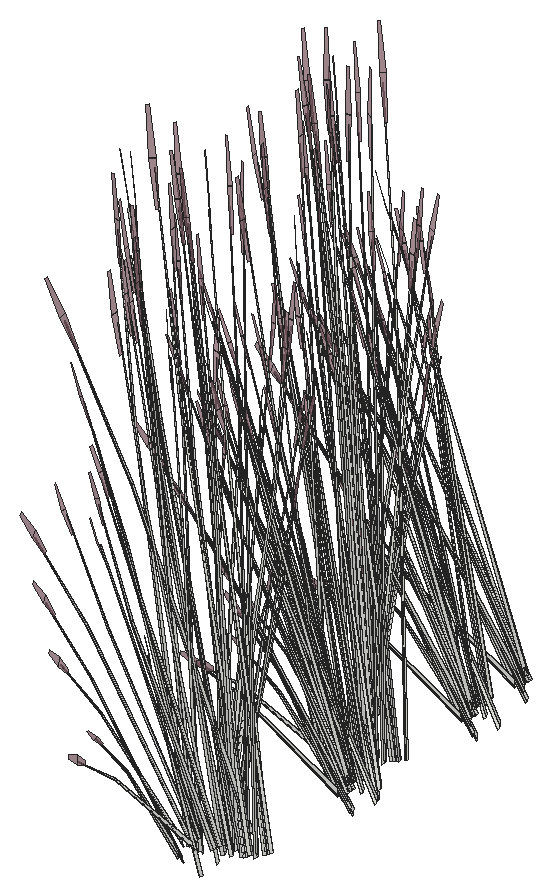
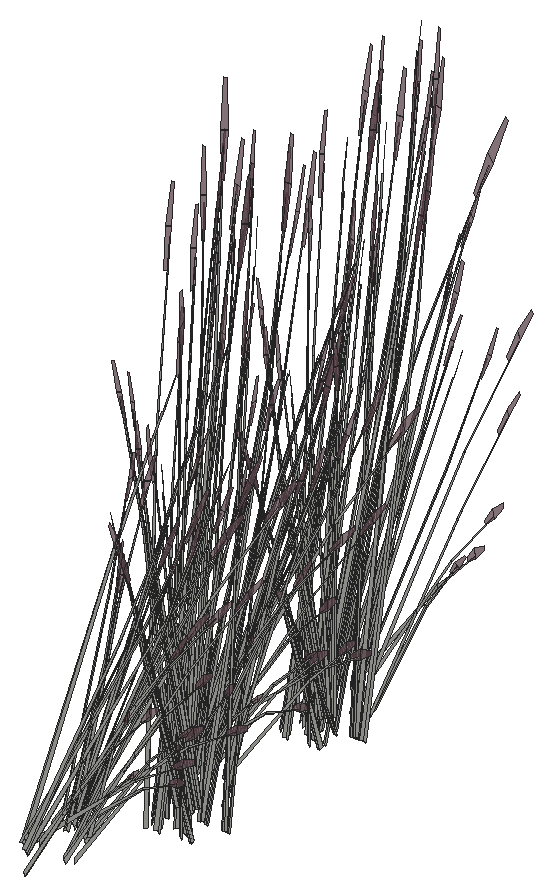
# SketchUp Ruby script. Lengths in inches.
U = 1.inch
M = Sketchup.active_model
def pt(a) = Geom::Point3d.new(a.map { |v| v * U })
def face(e, loops, mat)
  f = e.add_face(loops[0].map { |a| pt(a) })
  loops[1..].each { |l| e.add_face(l.map { |a| pt(a) }).erase! }
  f.material = f.back_material = mat if mat
  f
end
# faces: each face lists its corners as indices into pts; further lists are holes
def faces(e, pts, list, mat = nil) = list.each { |f| face(e, (f[0].is_a?(Array) ? f : [f]).map { |l| l.map { |i| pts[i] } }, mat) }
# xy, xz, yz: faces in a plane at the given z, y or x. An outline is a flat list of corners, or four numbers for a rectangle; further outlines are holes
def ring(l) = l.size == 4 ? [[l[0], l[1]], [l[2], l[1]], [l[2], l[3]], [l[0], l[3]]] : l.each_slice(2).to_a
def flat(e, list, mat, &to3) = list.each { |f| face(e, (f[0].is_a?(Array) ? f : [f]).map { |l| ring(l).map { |u, v| to3.(u, v) } }, mat) }
def xy(e, z, list, mat = nil) = flat(e, list, mat) { |x, y| [x, y, z] }
def xz(e, y, list, mat = nil) = flat(e, list, mat) { |x, z| [x, y, z] }
def yz(e, x, list, mat = nil) = flat(e, list, mat) { |y, z| [x, y, z] }
def lines(e, pts, list) = list.each { |a, b| e.add_line(pt(pts[a]), pt(pts[b])) }
# prism: a flat outline (further loops are holes) pulled along v
def prism(e, loops, v, mat = nil)
  f = face(e, loops, mat); d = Geom::Vector3d.new(v.map { |x| x * U })
  f.pushpull(f.normal.samedirection?(d) ? d.length : -d.length)
end
def box(e, o, s, mat = nil) = prism(e, [[o, [o[0] + s[0], o[1], o[2]], [o[0] + s[0], o[1] + s[1], o[2]], [o[0], o[1] + s[1], o[2]]]], [0, 0, s[2]], mat)
def at(x, y, z, deg = 0) = Geom::Transformation.translation(pt([x, y, z])) * Geom::Transformation.rotation(ORIGIN, Z_AXIS, deg.degrees)
def axes(o, x, y, z) = Geom::Transformation.new([*x, 0, *y, 0, *z, 0, *pt(o).to_a, 1])
def part(name) = M.definitions.add(name)
# library, detail: a bought-in or finely detailed component or shape, given as its bounding box
def library(name, o, s) = part(name).tap { |d| box(d.entities, o, s) }
def detail(e, o, s) = box(e.add_group.entities, o, s)
def put(e, d, t, mat = nil) = e.add_instance(d, t).tap { |i| i.material = mat if mat }
def group(e, t, mat = nil) = e.add_group.tap { |g| g.transformation = t; g.material = mat if mat }.entities
root = M.entities
M.materials.add("LightPink_Translucent").color = [144, 107, 117]
M.materials["LightPink_Translucent"].alpha = 0.75
c1 = part("blade")
p = [[2.15,0.21,22],[0,0.17,0],[0.09,0.45,0],[2.18,0.31,22],[2.29,0.31,22],[0.38,0.45,0],
  [2.48,0.24,33],[2.49,0.24,33],[2.48,0.22,33]]
faces(c1.entities,p,[[0,1,2,3],[4,5,2,3],[6,3,4,7],[8,0,3,6]])
c2 = part("seeds")
p = [[0.3,-0.1,1.38],[-0.01,-0.03,1.59],[-0.01,-0.03,0.03],[0.14,-0.07,-0.07],[0.29,-0.03,3],[0.15,0.01,3.11]]
faces(c2.entities,p,[[0,1,2,3],[1,0,4,5]],"LightPink_Translucent")
c3 = part("blade with seeds")
put(c3.entities,c1,at(0,0,0))
put(c3.entities,c2,axes([2.4,0.25,30.99],[1.5799,-0.05474,1.17369],[-0.12525,1.92788,0.29478],[-0.07173,-0.02425,1.56792]))
put(root,c3,axes([286.88,431.23,4.71],[-0.01669,0.07821,1.77383],[-0.82314,0.28383,-0.16761],[-0.24223,-0.14508,0.31391]))
put(root,c3,axes([284.46,454.61,5.34],[-0.02328,0.60353,-0.7886],[-0.98022,-0.04053,0.09517],[-0.10344,0.25568,1.11556]))
put(root,c3,axes([286,432.36,2.59],[-0.05417,0.21344,1.43002],[-0.79196,0.17867,-0.30754],[-0.18512,-0.27588,0.61141]))
put(root,c3,axes([289.62,448.64,2.59],[0.3109,0.05356,1.43002],[0.20038,0.54709,-0.30754],[-0.42231,0.10241,0.61141]))
put(root,c3,axes([284.45,456.3125,2.77],[-0.02315,-0.38796,1.1486],[0.57853,0.27671,0.84392],[-0.11378,0.18492,0.25299]))
put(root,c3,axes([289.64,463.32,2.59],[0.3109,0.05356,1.43002],[0.20038,0.54709,-0.30754],[-0.42231,0.10241,0.61141]))
put(root,c3,axes([285.26,449.68,5.09],[0.99656,-0.1677,0.53763],[0.17295,0.65785,0.4433],[-0.23438,-0.19388,1.11249]))
put(root,c3,axes([286.26,432.91,3.875],[0.2045,0.20949,1.71376],[-0.94495,0.17636,0.13857],[-0.21357,-0.32887,0.73262]))
put(root,c3,axes([288,436.41,2.67],[-0.90324,0.43318,-0.29095],[-0.60064,-0.61207,-0.50002],[-0.22285,-0.06216,1.59708]))
put(root,c3,axes([287.13,453.5625,2.21],[-0.97146,0.04028,-0.44739],[-0.08785,-0.66859,0.21531],[-0.17391,0.06776,1.43643]))
put(root,c3,axes([285.5,437.78,4.73],[-0.63704,-0.44518,0.48003],[0.67652,-0.38394,0.3958],[-0.11751,0.20886,0.9933]))
put(root,c3,axes([286.59,432.8,4.53],[-0.13817,-0.52554,-0.35414],[0.78985,-0.13877,0.4572],[-0.21215,-0.1506,0.87481]))
put(root,c3,axes([284.39,435.46,2.375],[-1.11865,0,0],[0,-0.72922,-0.51607],[0,-0.16609,1.63711]))
put(root,c3,axes([285.96,437.32,2.03],[-0.21015,-0.56852,-0.30978],[0.83462,-0.16144,0.30978],[-0.16826,-0.06556,1.38974]))
put(root,c3,axes([292.37,446.89,3.34],[0.25429,-0.09438,1.77064],[0.08769,0.65901,0.13857],[-0.5508,0.08745,0.63284]))
put(root,c3,axes([292.39,461.5625,3.34],[0.25429,-0.09438,1.77064],[0.08769,0.65901,0.13857],[-0.5508,0.08745,0.63284]))
put(root,c3,axes([285.49,449.82,4.73],[0.4066,-0.41448,0.0643],[0.57901,0.24131,0.50621],[-0.18719,-0.13288,0.77189]))
put(root,c3,axes([285.27,437.73,4.73],[-0.73517,-0.0304,0.0643],[0.02016,-0.45906,0.50621],[-0.07693,0.17585,0.77189]))
put(root,c3,axes([285.27,454.68,2.48],[0.83726,0.32623,0.49651],[-0.50045,0.58498,0],[-0.19069,-0.0743,1.57504]))
put(root,c3,axes([285.5,437.91,4.53],[-0.60531,0.34352,-0.35414],[-0.573,-0.39225,0.4572],[-0.08718,0.19929,0.87481]))
put(root,c3,axes([284.14,455.46,3.36],[0.01966,-0.33682,1.54345],[0.88405,0.17791,0.21329],[-0.0766,0.35897,0.72882]))
put(root,c3,axes([286.0625,453.48,2.4375],[0.23711,-0.77313,-0.23429],[1.12425,0.13477,0.51271],[-0.19645,-0.10677,1.5644]))
put(root,c3,axes([288.6,436.88,2.06],[-0.60257,0.49041,-0.62353],[-0.74854,-0.44469,-0.16365],[-0.24146,0.12234,1.37633]))
put(root,c3,axes([287.05,433.23,5.05],[0.13817,0.52554,0.35414],[-0.78985,0.13877,-0.4572],[-0.21215,-0.1506,0.87481]))
put(root,c3,axes([286.47,453.66,2.62],[-0.17258,0.58229,0.1448],[-0.84319,-0.10108,-0.41347],[-0.15345,-0.05979,1.26744]))
put(root,c3,axes([283.34,439.13,4.71],[0.10149,-0.03939,1.77383],[0.83886,0.26202,-0.16761],[-0.01971,0.21816,0.31391]))
put(root,c3,axes([291.46,467.01,4.98],[-0.89428,-0.01571,-0.71045],[0.06006,-0.66153,0.08574],[-0.37886,-0.06981,1.00501]))
put(root,c3,axes([286.375,448.59,4.72],[-0.13683,-0.09148,1.74944],[-0.91315,0.058,-0.27667],[-0.14574,-0.2188,0.14031]))
put(root,c3,axes([285.25,435.27,2.33],[-0.83213,0.54855,0.30756],[-0.83263,-0.54278,-0.36492],[-0.02906,-0.15578,1.64885]))
put(root,c3,axes([289.64,447.33,4.72],[-0.14609,0.08471,1.74944],[0.01243,0.61893,-0.27667],[-0.33486,0.08049,0.14031]))
put(root,c3,axes([288.15,455.29,2.02],[-0.83726,0.32623,-0.49651],[-0.50045,-0.58498,0],[-0.19069,0.0743,1.57504]))
put(root,c3,axes([289.66,462,4.72],[-0.14609,0.08471,1.74944],[0.01243,0.61893,-0.27667],[-0.33486,0.08049,0.14031]))
put(root,c3,axes([283.19,452.04,2.02],[0,-0.65246,-0.49651],[1.00089,0,0],[0,-0.1486,1.57504]))
put(root,c3,axes([291.55,445.83,4.98],[-0.89428,-0.01571,-0.71045],[0.06006,-0.66153,0.08574],[-0.37886,-0.06981,1.00501]))
put(root,c3,axes([283.62,452.64,2.48],[0,0.65246,0.49651],[-1.00089,0,0],[0,-0.1486,1.57504]))
put(root,c3,axes([291.5625,460.51,4.98],[-0.89428,-0.01571,-0.71045],[0.06006,-0.66153,0.08574],[-0.37886,-0.06981,1.00501]))
put(root,c3,axes([288.21,455.11,2.19],[-0.55235,-0.65609,-0.05142],[0.93577,-0.36461,0.51607],[-0.23059,0.06247,1.6363]))
put(root,c3,axes([290.74,467.17,2.59],[0.17466,0.18165,1.43002],[-0.40248,0.49377,-0.30754],[-0.41327,-0.11802,0.61141]))
put(root,c3,axes([288.68,436.79,3.33],[0.77308,0.2631,1.51261],[-0.75736,0.56681,0.59816],[-0.33924,-0.33594,1.26806]))
put(root,c3,axes([290.82,445.99,2.59],[0.17466,0.18165,1.43002],[-0.40248,0.49377,-0.30754],[-0.41327,-0.11802,0.61141]))
put(root,c3,axes([290.84,460.67,2.59],[0.17466,0.18165,1.43002],[-0.40248,0.49377,-0.30754],[-0.41327,-0.11802,0.61141]))
put(root,c3,axes([285.73,432.02,2.77],[0.46666,0.22709,1.1486],[-0.67962,0.13651,0.84392],[-0.14541,-0.17452,0.25299]))
put(root,c3,axes([291.06,466.58,3.875],[0.3323,0.11241,1.71376],[-0.68769,0.4716,0.13857],[-0.42861,-0.21275,0.73262]))
put(root,c3,axes([289.01,436.61,2.46],[-0.87356,-0.52515,-0.25192],[0.73507,-0.5897,0.5513],[-0.23523,0.06143,1.68216]))
put(root,c3,axes([290.11,446.98,4.53],[-0.74348,-0.18202,-0.35414],[0.21685,-0.53102,0.4572],[-0.29933,0.04869,0.87481]))
put(root,c3,axes([287.43,436.1,2.21],[-0.53742,-0.54764,-0.44739],[0.81403,-0.38564,0.21531],[-0.17391,-0.06776,1.43643]))
put(root,c3,axes([290.13,461.65,4.53],[-0.74348,-0.18202,-0.35414],[0.21685,-0.53102,0.4572],[-0.29933,0.04869,0.87481]))
put(root,c3,axes([284.66,454.81,5],[0.64041,0.4384,-0.5672],[-0.67652,0.38394,-0.43934],[-0.09744,0.22274,1.08528]))
put(root,c3,axes([291.14,445.4,3.875],[0.3323,0.11241,1.71376],[-0.68769,0.4716,0.13857],[-0.42861,-0.21275,0.73262]))
put(root,c3,axes([291.16,460.07,3.875],[0.3323,0.11241,1.71376],[-0.68769,0.4716,0.13857],[-0.42861,-0.21275,0.73262]))
put(root,c3,axes([287.95,455.03,2.03],[-0.83462,-0.16144,-0.30978],[0.21015,-0.56852,0.30978],[-0.16826,0.06556,1.38974]))
put(root,c3,axes([284.375,454.49,5.05],[0.60531,-0.34352,0.35414],[0.573,0.39225,-0.4572],[-0.08718,0.19929,0.87481]))
put(root,c3,axes([285.91,437.55,5.34],[-0.02328,0.60353,-0.7886],[-0.98022,-0.04053,0.09517],[-0.10344,0.25568,1.11556]))
put(root,c3,axes([285.81,452.79,2.67],[-1.00749,-0.31132,-0.29095],[0.48511,-0.65709,-0.50002],[-0.03166,-0.16133,1.59708]))
put(root,c3,axes([288.43,452.6,2.84],[-0.02444,-0.61432,1.41272],[1.10603,0.15924,0.59816],[-0.26159,0.33615,1.3335]))
put(root,c3,axes([285.89,439.25,2.77],[-0.02315,-0.38796,1.1486],[0.57853,0.27671,0.84392],[-0.11378,0.18492,0.25299]))
put(root,c3,axes([286.7,432.61,5.09],[0.99656,-0.1677,0.53763],[0.17295,0.65785,0.4433],[-0.23438,-0.19388,1.11249]))
put(root,c3,axes([288.57,436.49,2.21],[-0.97146,0.04028,-0.44739],[-0.08785,-0.66859,0.21531],[-0.17391,0.06776,1.43643]))
put(root,c3,axes([288.02,447.96,4.71],[0.11417,0.0175,1.77383],[0.35319,0.57649,-0.16761],[-0.23371,0.15131,0.31391]))
put(root,c3,axes([290.62,447.25,4.68],[-0.24236,0.59349,-0.51099],[-0.83094,-0.20343,-0.3958],[-0.33455,0.05442,0.97773]))
put(root,c3,axes([288.03,462.63,4.71],[0.11417,0.0175,1.77383],[0.35319,0.57649,-0.16761],[-0.23371,0.15131,0.31391]))
put(root,c3,axes([290.64,461.92,4.68],[-0.24236,0.59349,-0.51099],[-0.83094,-0.20343,-0.3958],[-0.33455,0.05442,0.97773]))
put(root,c3,axes([291.17,467.15,4.68],[-0.6496,0.4322,-0.51099],[-0.5689,-0.45657,-0.3958],[-0.33005,-0.06576,0.97773]))
put(root,c3,axes([283.99,454.58,5.4],[0.98321,0.03233,-0.13498],[-0.02687,0.61208,-0.74919],[-0.0683,0.23574,1.13838]))
put(root,c3,axes([291.25,445.97,4.68],[-0.6496,0.4322,-0.51099],[-0.5689,-0.45657,-0.3958],[-0.33005,-0.06576,0.97773]))
put(root,c3,axes([291.27,460.64,4.68],[-0.6496,0.4322,-0.51099],[-0.5689,-0.45657,-0.3958],[-0.33005,-0.06576,0.97773]))
put(root,c3,axes([283.97,455.47,2.82],[0.8127,-0.11554,0.06507],[0.18684,0.46549,-0.86304],[-0.05152,0.23564,0.7736]))
put(root,c3,axes([286.93,432.76,4.73],[0.4066,-0.41448,0.0643],[0.57901,0.24131,0.50621],[-0.18719,-0.13288,0.77189]))
put(root,c3,axes([290.2,447.21,1.49],[0.02269,0.10283,1.76342],[-0.45738,0.53699,-0.26939],[-0.32488,-0.02707,0.30037]))
put(root,c3,axes([287.8125,453.38,2.67],[0.10425,0.7445,-0.29095],[-1.08575,0.04502,-0.50002],[-0.19119,0.09917,1.59708]))
put(root,c3,axes([290.22,461.89,1.49],[0.02269,0.10283,1.76342],[-0.45738,0.53699,-0.26939],[-0.32488,-0.02707,0.30037]))
put(root,c3,axes([285.36,452.13,2.1],[-0.36739,-0.66907,-0.69835],[1.05831,-0.24096,-0.18329],[-0.04061,-0.22656,1.54149]))
put(root,c3,axes([287.77,450,5.03],[-0.87543,0.30377,-0.1216],[-0.4302,-0.53915,-0.67495],[-0.1155,-0.2272,1.02557]))
put(root,c3,axes([287.01,450.03,4.68],[-0.87941,-0.16356,-0.51099],[0.30143,-0.56078,-0.3958],[-0.08064,-0.22578,0.97773]))
put(root,c3,axes([286.72,437.61,2.48],[0.83726,0.32623,0.49651],[-0.50045,0.58498,0],[-0.19069,-0.0743,1.57504]))
put(root,c3,axes([285.58,438.4,3.36],[0.01966,-0.33682,1.54345],[0.88405,0.17791,0.21329],[-0.0766,0.35897,0.72882]))
put(root,c3,axes([290.25,465.9375,4.71],[0.06632,0.06511,1.77383],[-0.31973,0.58531,-0.16761],[-0.32381,0.00424,0.31391]))
put(root,c3,axes([285.39,454.1875,3.875],[-0.0219,-0.25042,1.71376],[0.94901,0.16613,0.13857],[-0.0587,0.35688,0.73262]))
put(root,c3,axes([290.33,444.75,4.71],[0.06632,0.06511,1.77383],[-0.31973,0.58531,-0.16761],[-0.32381,0.00424,0.31391]))
put(root,c3,axes([290.35,459.43,4.71],[0.06632,0.06511,1.77383],[-0.31973,0.58531,-0.16761],[-0.32381,0.00424,0.31391]))
put(root,c3,axes([287.51,436.42,2.4375],[0.23711,-0.77313,-0.23429],[1.12425,0.13477,0.51271],[-0.19645,-0.10677,1.5644]))
put(root,c3,axes([283.62,452.05,2.03],[0.62448,-0.40708,-0.30978],[0.62448,0.40708,0.30978],[0,-0.13112,1.38974]))
put(root,c3,axes([288.97,449.79,2.77],[0.37283,-0.29571,1.1486],[0.14711,0.46813,0.84392],[-0.26943,0.08382,0.25299]))
put(root,c3,axes([290.99,465.55,4.72],[-0.19249,-0.00461,1.74944],[-0.61281,0.46055,-0.27667],[-0.32697,-0.0941,0.14031]))
put(root,c3,axes([288.99,464.46,2.77],[0.37283,-0.29571,1.1486],[0.14711,0.46813,0.84392],[-0.26943,0.08382,0.25299]))
put(root,c3,axes([286.44,449.42,2.13],[-0.61821,0.37431,-0.03893],[-0.56645,-0.40995,-0.17649],[-0.03988,-0.11616,0.58215]))
put(root,c3,axes([287.91,436.6,2.62],[-0.17258,0.58229,0.1448],[-0.84319,-0.10108,-0.41347],[-0.15345,-0.05979,1.26744]))
put(root,c3,axes([291.07,444.36,4.72],[-0.19249,-0.00461,1.74944],[-0.61281,0.46055,-0.27667],[-0.32697,-0.0941,0.14031]))
put(root,c3,axes([291.09,459.04,4.72],[-0.19249,-0.00461,1.74944],[-0.61281,0.46055,-0.27667],[-0.32697,-0.0941,0.14031]))
put(root,c3,axes([286.19,453.11,2.36],[1.13071,0.13747,0.45755],[-0.23011,0.77639,0.17955],[-0.16524,-0.07497,1.58856]))
put(root,c3,axes([287.82,431.52,4.72],[-0.13683,-0.09148,1.74944],[-0.91315,0.058,-0.27667],[-0.14574,-0.2188,0.14031]))
put(root,c3,axes([289.59,438.22,2.02],[-0.83726,0.32623,-0.49651],[-0.50045,-0.58498,0],[-0.19069,0.0743,1.57504]))
put(root,c3,axes([284.64,434.97,2.02],[0,-0.65246,-0.49651],[1.00089,0,0],[0,-0.1486,1.57504]))
put(root,c3,axes([285.06,435.58,2.48],[0,0.65246,0.49651],[-1.00089,0,0],[0,-0.1486,1.57504]))
put(root,c3,axes([289.65,438.05,2.19],[-0.55235,-0.65609,-0.05142],[0.93577,-0.36461,0.51607],[-0.23059,0.06247,1.6363]))
put(root,c3,axes([290.28,446.91,4.73],[0.25275,-0.59491,0.48003],[0.83094,0.20343,0.3958],[-0.32677,0.03575,0.9933]))
put(root,c3,axes([290.3,461.59,4.73],[0.25275,-0.59491,0.48003],[0.83094,0.20343,0.3958],[-0.32677,0.03575,0.9933]))
put(root,c3,axes([290.93,466.74,4.53],[-0.50902,-0.40851,-0.35414],[0.58122,-0.38671,0.4572],[-0.29531,-0.05884,0.87481]))
put(root,c3,axes([290.58,446.74,5.03],[0.45012,0.59081,-0.1216],[-0.79888,0.29033,-0.67495],[-0.33665,0.07795,1.02557]))
put(root,c3,axes([290.6,461.41,5.03],[0.45012,0.59081,-0.1216],[-0.79888,0.29033,-0.67495],[-0.33665,0.07795,1.02557]))
put(root,c3,axes([291.59,445.51,5.03],[-0.0479,0.66354,-0.1216],[-0.90696,-0.01814,-0.67495],[-0.3493,-0.04609,1.02557]))
put(root,c3,axes([291.61,460.1875,5.03],[-0.0479,0.66354,-0.1216],[-0.90696,-0.01814,-0.67495],[-0.3493,-0.04609,1.02557]))
put(root,c3,axes([291.01,445.56,4.53],[-0.50902,-0.40851,-0.35414],[0.58122,-0.38671,0.4572],[-0.29531,-0.05884,0.87481]))
put(root,c3,axes([291.03,460.23,4.53],[-0.50902,-0.40851,-0.35414],[0.58122,-0.38671,0.4572],[-0.29531,-0.05884,0.87481]))
put(root,c3,axes([290.22,446.75,4.73],[-0.32857,-0.44488,0.0643],[0.59916,-0.21775,0.50621],[-0.26412,0.04296,0.77189]))
put(root,c3,axes([285.9,452.97,2.72],[-0.43405,0.58792,0.44739],[-0.90188,-0.28295,-0.21531],[0,-0.13553,1.43643]))
put(root,c3,axes([287.33,450.14,4.98],[-0.42698,-0.53052,-0.71045],[0.87893,-0.29566,0.08574],[-0.09984,-0.25633,1.00501]))
put(root,c3,axes([290.24,461.43,4.73],[-0.32857,-0.44488,0.0643],[0.59916,-0.21775,0.50621],[-0.26412,0.04296,0.77189]))
put(root,c3,axes([286.1,437.75,5],[0.64041,0.4384,-0.5672],[-0.67652,0.38394,-0.43934],[-0.09744,0.22274,1.08528]))
put(root,c3,axes([291.73,447.98,3.875],[0.22344,-0.20048,1.71376],[0.56419,0.54113,0.13857],[-0.38697,0.24643,0.73262]))
put(root,c3,axes([290.38,448.51,4.53],[-0.77872,0.09325,-0.35414],[-0.20563,-0.53305,0.4572],[-0.22316,0.14318,0.87481]))
put(root,c3,axes([289.4,437.96,2.03],[-0.83462,-0.16144,-0.30978],[0.21015,-0.56852,0.30978],[-0.16826,0.06556,1.38974]))
put(root,c3,axes([290.4,463.18,4.53],[-0.77872,0.09325,-0.35414],[-0.20563,-0.53305,0.4572],[-0.22316,0.14318,0.87481]))
put(root,c3,axes([285.82,437.42,5.05],[0.60531,-0.34352,0.35414],[0.573,0.39225,-0.4572],[-0.08718,0.19929,0.87481]))
put(root,c3,axes([287.25,435.72,2.67],[-1.00749,-0.31132,-0.29095],[0.48511,-0.65709,-0.50002],[-0.03166,-0.16133,1.59708]))
put(root,c3,axes([289.875,435.53,2.84],[-0.02444,-0.61432,1.41272],[1.10603,0.15924,0.59816],[-0.26159,0.33615,1.3335]))
put(root,c3,axes([289.96,450.09,1.49],[0.12,0.06519,1.76342],[0.20347,0.60397,-0.26939],[-0.26596,0.12879,0.30037]))
put(root,c3,axes([289.78,446.54,2.77],[0.57115,-0.04669,1.1486],[-0.36229,0.41137,0.84392],[-0.28224,-0.06171,0.25299]))
put(root,c3,axes([289.8,461.21,2.77],[0.57115,-0.04669,1.1486],[-0.36229,0.41137,0.84392],[-0.28224,-0.06171,0.25299]))
put(root,c3,axes([285.59,454.35,2.47],[0.96132,-0.17317,0.17642],[0.23737,0.64447,0.35086],[-0.08574,-0.0939,1.60407]))
put(root,c3,axes([285.43,437.52,5.4],[0.98321,0.03233,-0.13498],[-0.02687,0.61208,-0.74919],[-0.0683,0.23574,1.13838]))
put(root,c3,axes([286.82,454.45,2.2],[-0.90188,-0.29293,0],[0.43405,-0.60866,0],[0,0,1.62707]))
put(root,c3,axes([287.5,450.21,5.05],[-0.2697,0.50175,0.35414],[-0.78684,-0.14635,-0.4572],[-0.07215,-0.20201,0.87481]))
put(root,c3,axes([288.91,455.1875,2.375],[0.55932,0.6538,0],[-0.93577,0.36461,-0.51607],[-0.21313,0.08304,1.63711]))
put(root,c3,axes([285.41,438.41,2.82],[0.8127,-0.11554,0.06507],[0.18684,0.46549,-0.86304],[-0.05152,0.23564,0.7736]))
put(root,c3,axes([290.48,448.39,4.73],[-0.22187,-0.60049,0.48003],[0.87033,-0.10422,0.3958],[-0.25651,0.14123,0.9933]))
put(root,c3,axes([290.5,463.07,4.73],[-0.22187,-0.60049,0.48003],[0.87033,-0.10422,0.3958],[-0.25651,0.14123,0.9933]))
put(root,c3,axes([289.25,436.3125,2.67],[0.10425,0.7445,-0.29095],[-1.08575,0.04502,-0.50002],[-0.19119,0.09917,1.59708]))
put(root,c3,axes([286.8,435.0625,2.1],[-0.36739,-0.66907,-0.69835],[1.05831,-0.24096,-0.18329],[-0.04061,-0.22656,1.54149]))
put(root,c3,axes([289.21,432.9375,5.03],[-0.87543,0.30377,-0.1216],[-0.4302,-0.53915,-0.67495],[-0.1155,-0.2272,1.02557]))
put(root,c3,axes([290.85,466.59,5.09],[0.7388,-0.48151,0.53763],[0.63717,0.51135,0.4433],[-0.34662,-0.08882,1.11249]))
put(root,c3,axes([288.46,432.96,4.68],[-0.87941,-0.16356,-0.51099],[0.30143,-0.56078,-0.3958],[-0.08064,-0.22578,0.97773]))
put(root,c3,axes([286.0625,455.47,5.0625],[-0.88151,-0.17057,0.53283],[0.30143,-0.56078,0.43934],[0.05297,0.22053,1.10256]))
put(root,c3,axes([290.93,445.41,5.09],[0.7388,-0.48151,0.53763],[0.63717,0.51135,0.4433],[-0.34662,-0.08882,1.11249]))
put(root,c3,axes([290.95,460.08,5.09],[0.7388,-0.48151,0.53763],[0.63717,0.51135,0.4433],[-0.34662,-0.08882,1.11249]))
put(root,c3,axes([290.31,448.28,4.73],[-0.61415,-0.2744,0.0643],[0.35756,-0.39076,0.50621],[-0.1969,0.12633,0.77189]))
put(root,c3,axes([286.83,437.12,3.875],[-0.0219,-0.25042,1.71376],[0.94901,0.16613,0.13857],[-0.0587,0.35688,0.73262]))
put(root,c3,axes([290.33,462.95,4.73],[-0.61415,-0.2744,0.0643],[0.35756,-0.39076,0.50621],[-0.1969,0.12633,0.77189]))
put(root,c3,axes([285.83,455.51,4.73],[-0.6592,0.22175,0.0643],[-0.32265,-0.40436,0.50621],[0.06366,0.17825,0.77189]))
put(root,c3,axes([288.45,454.39,2.47],[0.25843,-0.64844,0.17642],[0.9457,0.1835,0.35086],[-0.16336,0.00316,1.60407]))
put(root,c3,axes([288.01,453.53,2.62],[0.66093,0.39201,0.1448],[-0.5513,0.44227,-0.41347],[-0.15345,0.05979,1.26744]))
put(root,c3,axes([285.06,434.98,2.03],[0.62448,-0.40708,-0.30978],[0.62448,0.40708,0.30978],[0,-0.13112,1.38974]))
put(root,c3,axes([287.88,432.35,2.13],[-0.61821,0.37431,-0.03893],[-0.56645,-0.40995,-0.17649],[-0.03988,-0.11616,0.58215]))
put(root,c3,axes([287.78,453.04,2.3],[-0.83213,-0.56158,-0.06131],[0.83263,-0.56193,0],[-0.02906,-0.01961,1.75571]))
put(root,c3,axes([287.64,436.04,2.36],[1.13071,0.13747,0.45755],[-0.23011,0.77639,0.17955],[-0.16524,-0.07497,1.58856]))
